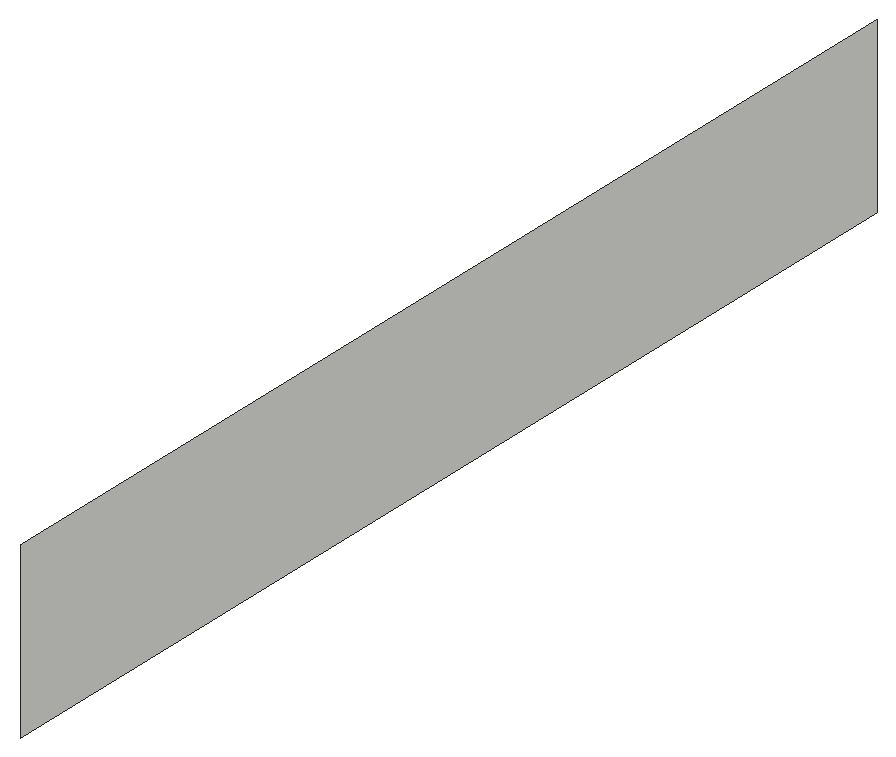
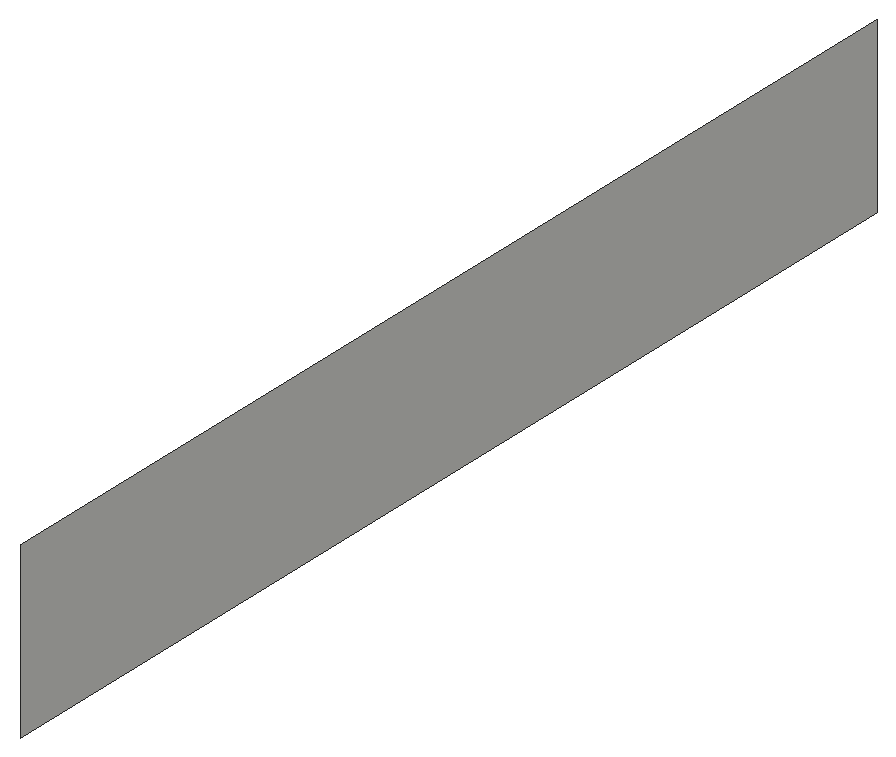
# SketchUp Ruby script. Lengths in inches.
U = 1.inch
M = Sketchup.active_model
def pt(a) = Geom::Point3d.new(a.map { |v| v * U })
def face(e, loops, mat)
  f = e.add_face(loops[0].map { |a| pt(a) })
  loops[1..].each { |l| e.add_face(l.map { |a| pt(a) }).erase! }
  f.material = f.back_material = mat if mat
  f
end
# faces: each face lists its corners as indices into pts; further lists are holes
def faces(e, pts, list, mat = nil) = list.each { |f| face(e, (f[0].is_a?(Array) ? f : [f]).map { |l| l.map { |i| pts[i] } }, mat) }
# xy, xz, yz: faces in a plane at the given z, y or x. An outline is a flat list of corners, or four numbers for a rectangle; further outlines are holes
def ring(l) = l.size == 4 ? [[l[0], l[1]], [l[2], l[1]], [l[2], l[3]], [l[0], l[3]]] : l.each_slice(2).to_a
def flat(e, list, mat, &to3) = list.each { |f| face(e, (f[0].is_a?(Array) ? f : [f]).map { |l| ring(l).map { |u, v| to3.(u, v) } }, mat) }
def xy(e, z, list, mat = nil) = flat(e, list, mat) { |x, y| [x, y, z] }
def xz(e, y, list, mat = nil) = flat(e, list, mat) { |x, z| [x, y, z] }
def yz(e, x, list, mat = nil) = flat(e, list, mat) { |y, z| [x, y, z] }
def lines(e, pts, list) = list.each { |a, b| e.add_line(pt(pts[a]), pt(pts[b])) }
# prism: a flat outline (further loops are holes) pulled along v
def prism(e, loops, v, mat = nil)
  f = face(e, loops, mat); d = Geom::Vector3d.new(v.map { |x| x * U })
  f.pushpull(f.normal.samedirection?(d) ? d.length : -d.length)
end
def box(e, o, s, mat = nil) = prism(e, [[o, [o[0] + s[0], o[1], o[2]], [o[0] + s[0], o[1] + s[1], o[2]], [o[0], o[1] + s[1], o[2]]]], [0, 0, s[2]], mat)
def at(x, y, z, deg = 0) = Geom::Transformation.translation(pt([x, y, z])) * Geom::Transformation.rotation(ORIGIN, Z_AXIS, deg.degrees)
def axes(o, x, y, z) = Geom::Transformation.new([*x, 0, *y, 0, *z, 0, *pt(o).to_a, 1])
def part(name) = M.definitions.add(name)
# library, detail: a bought-in or finely detailed component or shape, given as its bounding box
def library(name, o, s) = part(name).tap { |d| box(d.entities, o, s) }
def detail(e, o, s) = box(e.add_group.entities, o, s)
def put(e, d, t, mat = nil) = e.add_instance(d, t).tap { |i| i.material = mat if mat }
def group(e, t, mat = nil) = e.add_group.tap { |g| g.transformation = t; g.material = mat if mat }.entities
root = M.entities
yz(root,277.93,[[198.23,92.87,221.48,96.63]])
